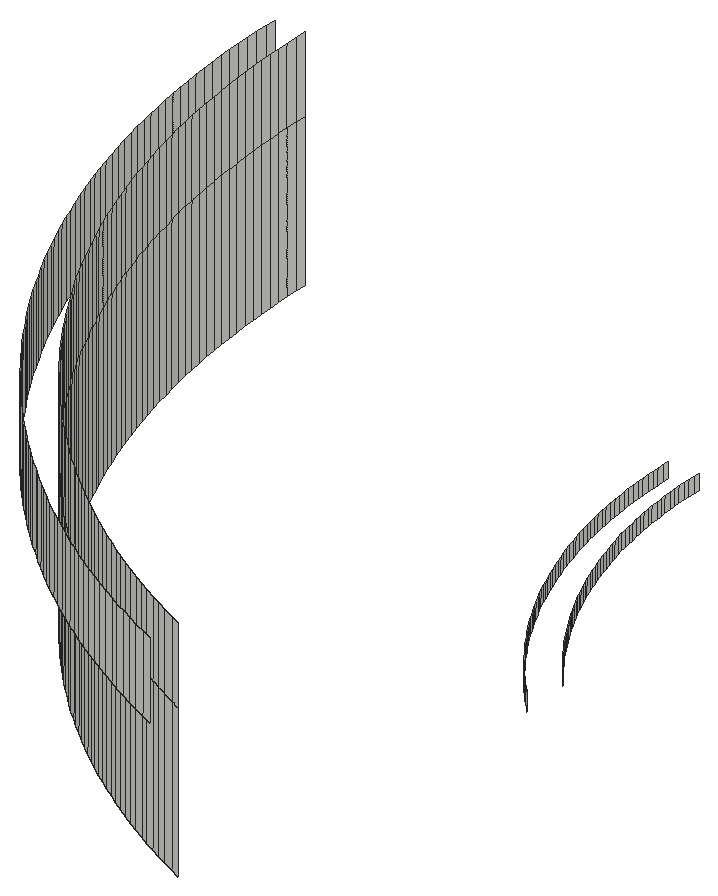
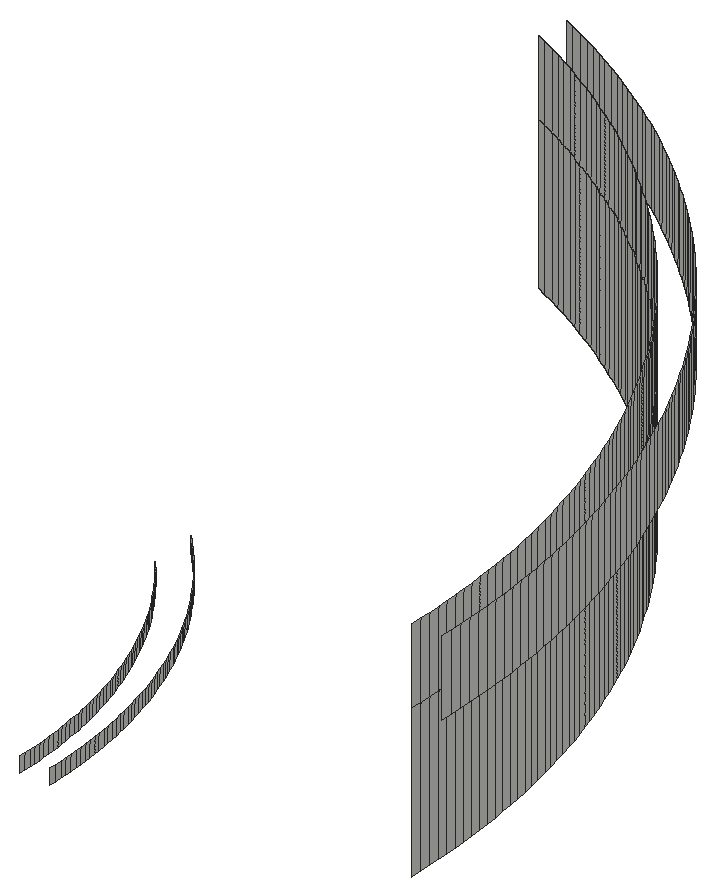
# SketchUp Ruby script. Lengths in inches.
U = 1.inch
M = Sketchup.active_model
def pt(a) = Geom::Point3d.new(a.map { |v| v * U })
def face(e, loops, mat)
  f = e.add_face(loops[0].map { |a| pt(a) })
  loops[1..].each { |l| e.add_face(l.map { |a| pt(a) }).erase! }
  f.material = f.back_material = mat if mat
  f
end
# faces: each face lists its corners as indices into pts; further lists are holes
def faces(e, pts, list, mat = nil) = list.each { |f| face(e, (f[0].is_a?(Array) ? f : [f]).map { |l| l.map { |i| pts[i] } }, mat) }
# xy, xz, yz: faces in a plane at the given z, y or x. An outline is a flat list of corners, or four numbers for a rectangle; further outlines are holes
def ring(l) = l.size == 4 ? [[l[0], l[1]], [l[2], l[1]], [l[2], l[3]], [l[0], l[3]]] : l.each_slice(2).to_a
def flat(e, list, mat, &to3) = list.each { |f| face(e, (f[0].is_a?(Array) ? f : [f]).map { |l| ring(l).map { |u, v| to3.(u, v) } }, mat) }
def xy(e, z, list, mat = nil) = flat(e, list, mat) { |x, y| [x, y, z] }
def xz(e, y, list, mat = nil) = flat(e, list, mat) { |x, z| [x, y, z] }
def yz(e, x, list, mat = nil) = flat(e, list, mat) { |y, z| [x, y, z] }
def lines(e, pts, list) = list.each { |a, b| e.add_line(pt(pts[a]), pt(pts[b])) }
# prism: a flat outline (further loops are holes) pulled along v
def prism(e, loops, v, mat = nil)
  f = face(e, loops, mat); d = Geom::Vector3d.new(v.map { |x| x * U })
  f.pushpull(f.normal.samedirection?(d) ? d.length : -d.length)
end
def box(e, o, s, mat = nil) = prism(e, [[o, [o[0] + s[0], o[1], o[2]], [o[0] + s[0], o[1] + s[1], o[2]], [o[0], o[1] + s[1], o[2]]]], [0, 0, s[2]], mat)
def at(x, y, z, deg = 0) = Geom::Transformation.translation(pt([x, y, z])) * Geom::Transformation.rotation(ORIGIN, Z_AXIS, deg.degrees)
def axes(o, x, y, z) = Geom::Transformation.new([*x, 0, *y, 0, *z, 0, *pt(o).to_a, 1])
def part(name) = M.definitions.add(name)
# library, detail: a bought-in or finely detailed component or shape, given as its bounding box
def library(name, o, s) = part(name).tap { |d| box(d.entities, o, s) }
def detail(e, o, s) = box(e.add_group.entities, o, s)
def put(e, d, t, mat = nil) = e.add_instance(d, t).tap { |i| i.material = mat if mat }
def group(e, t, mat = nil) = e.add_group.tap { |g| g.transformation = t; g.material = mat if mat }.entities
root = M.entities
yz(root,9,[[233.61,354.5,234,357]])
yz(root,10,[[233.62,349.5,234,354.5],[233.62,354.5,234,357]])
yz(root,22,[[233.78,348,234,348.5]])
yz(root,22.01,[[233.33,348,233.55,348.5]])
yz(root,23,[[233.79,348,234,348.5]])
yz(root,23.01,[[233.37,348,233.58,348.5]])
p = [[26.82,222.14,348],[26.67,222.3,348],[26.67,222.3,348.5],[26.82,222.14,348.5],[26.52,222.46,348],[26.52,222.46,348.5],
  [26.37,222.625,348],[26.37,222.625,348.5],[26.22,222.79,348],[26.22,222.79,348.5],[26.07,222.96,348],[26.07,222.96,348.5],
  [25.93,223.13,348],[25.93,223.13,348.5],[25.79,223.3,348],[25.79,223.3,348.5],[25.65,223.48,348],[25.65,223.48,348.5],
  [25.51,223.65,348],[25.51,223.65,348.5],[25.38,223.83,348],[25.38,223.83,348.5],[25.25,224.01,348],[25.25,224.01,348.5],
  [26.57,223.93,348],[26.7,223.77,348],[26.7,223.77,348.5],[26.57,223.93,348.5],[26.43,224.09,348],[26.43,224.09,348.5],
  [25.12,224.1875,348],[25.12,224.1875,348.5],[26.31,224.26,348],[26.31,224.26,348.5],[24.99,224.37,348],[24.99,224.37,348.5],
  [26.18,224.43,348],[26.18,224.43,348.5],[24.87,224.56,348],[24.87,224.56,348.5],[26.06,224.6,348],[26.06,224.6,348.5],
  [24.74,224.74,348],[24.74,224.74,348.5],[25.93,224.77,348],[25.93,224.77,348.5],[24.62,224.93,348],[24.62,224.93,348.5],
  [25.8125,224.9375,348],[25.8125,224.9375,348.5],[24.51,225.12,348],[24.51,225.12,348.5],[25.7,225.11,348],[25.7,225.11,348.5],
  [24.39,225.31,348],[24.39,225.31,348.5],[25.58,225.29,348],[25.58,225.29,348.5],[24.28,225.5,348],[24.28,225.5,348.5],
  [25.47,225.46,348],[25.47,225.46,348.5],[24.17,225.69,348],[24.17,225.69,348.5],[25.36,225.64,348],[25.36,225.64,348.5],
  [25.25,225.82,348],[25.25,225.82,348.5],[24.06,225.89,348],[24.06,225.89,348.5],[25.14,226,348],[25.14,226,348.5],
  [23.96,226.08,348],[23.96,226.08,348.5],[25.04,226.18,348],[25.04,226.18,348.5],[23.85,226.28,348],[23.85,226.28,348.5],
  [24.9375,226.37,348],[24.9375,226.37,348.5],[23.75,226.48,348],[23.75,226.48,348.5],[24.84,226.55,348],[24.84,226.55,348.5],
  [23.66,226.68,348],[23.66,226.68,348.5],[24.74,226.74,348],[24.74,226.74,348.5],[23.5625,226.88,348],[23.5625,226.88,348.5],
  [24.65,226.92,348],[24.65,226.92,348.5],[23.47,227.09,348],[23.47,227.09,348.5],[24.56,227.11,348],[24.56,227.11,348.5],
  [23.38,227.29,348],[23.38,227.29,348.5],[24.47,227.3,348],[24.47,227.3,348.5],[23.29,227.49,348],[23.29,227.49,348.5],
  [24.38,227.49,348],[24.38,227.49,348.5],[23.21,227.7,348],[23.21,227.7,348.5],[24.3,227.68,348],[24.3,227.68,348.5],
  [23.13,227.91,348],[23.13,227.91,348.5],[24.22,227.88,348],[24.22,227.88,348.5],[23.05,228.12,348],[23.05,228.12,348.5],
  [24.14,228.07,348],[24.14,228.07,348.5],[22.98,228.33,348],[22.98,228.33,348.5],[24.0625,228.27,348],[24.0625,228.27,348.5],
  [22.9,228.54,348],[22.9,228.54,348.5],[23.99,228.46,348],[23.99,228.46,348.5],[22.83,228.75,348],[22.83,228.75,348.5],
  [23.92,228.66,348],[23.92,228.66,348.5],[22.76,228.96,348],[22.76,228.96,348.5],[23.85,228.86,348],[23.85,228.86,348.5],
  [23.78,229.06,348],[23.78,229.06,348.5],[22.7,229.17,348],[22.7,229.17,348.5],[23.72,229.26,348],[23.72,229.26,348.5],
  [22.64,229.39,348],[22.64,229.39,348.5],[23.66,229.46,348],[23.66,229.46,348.5],[22.58,229.6,348],[22.58,229.6,348.5],
  [23.6,229.66,348],[23.6,229.66,348.5],[22.52,229.82,348],[22.52,229.82,348.5],[23.55,229.86,348],[23.55,229.86,348.5],
  [22.47,230.03,348],[22.47,230.03,348.5],[23.49,230.0625,348],[23.49,230.0625,348.5],[22.42,230.25,348],[22.42,230.25,348.5],
  [23.44,230.26,348],[23.44,230.26,348.5],[22.37,230.47,348],[22.37,230.47,348.5],[23.39,230.47,348],[23.39,230.47,348.5],
  [22.33,230.68,348],[22.33,230.68,348.5],[23.35,230.67,348],[23.35,230.67,348.5],[22.28,230.9,348],[22.28,230.9,348.5],
  [23.31,230.88,348],[23.31,230.88,348.5],[22.25,231.12,348],[22.25,231.12,348.5],[23.27,231.08,348],[23.27,231.08,348.5],
  [22.21,231.34,348],[22.21,231.34,348.5],[23.23,231.29,348],[23.23,231.29,348.5],[22.18,231.5625,348],[22.18,231.5625,348.5],
  [23.2,231.5,348],[23.2,231.5,348.5],[23.17,231.7,348],[23.17,231.7,348.5],[22.15,231.78,348],[22.15,231.78,348.5],
  [23.14,231.91,348],[23.14,231.91,348.5],[22.12,232,348],[22.12,232,348.5],[23.11,232.12,348],[23.11,232.12,348.5],
  [22.09,232.22,348],[22.09,232.22,348.5],[23.09,232.33,348],[23.09,232.33,348.5],[22.07,232.44,348],[22.07,232.44,348.5],
  [23.07,232.54,348],[23.07,232.54,348.5],[22.05,232.67,348],[22.05,232.67,348.5],[23.05,232.74,348],[23.05,232.74,348.5],
  [22.04,232.89,348],[22.04,232.89,348.5],[23.03,232.95,348],[23.03,232.95,348.5],[22.02,233.11,348],[22.02,233.11,348.5],
  [23.02,233.16,348],[23.02,233.16,348.5],[22.01,233.33,348],[22.01,233.33,348.5],[23.01,233.37,348],[23.01,233.37,348.5],
  [22.01,233.55,348],[22,233.78,348],[22,233.78,348.5],[22.01,233.55,348.5],[23,233.79,348],[23.01,233.58,348],
  [23.01,233.58,348.5],[23,233.79,348.5],[26.52,207.83,349.5],[26.86,207.66,349.5],[26.86,207.66,354.5],[26.52,207.83,354.5],
  [26.17,207.99,349.5],[26.17,207.99,354.5],[25.83,208.16,349.5],[25.83,208.16,354.5],[25.5,208.34,349.5],[25.5,208.34,354.5],
  [25.16,208.51,349.5],[25.16,208.51,354.5],[24.83,208.7,349.5],[24.83,208.7,354.5],[24.5,208.89,349.5],[24.5,208.89,354.5],
  [24.17,209.08,349.5],[24.17,209.08,354.5],[23.85,209.27,349.5],[23.85,209.27,354.5],[23.53,209.47,349.5],[23.53,209.47,354.5],
  [23.21,209.68,349.5],[23.21,209.68,354.5],[22.89,209.89,349.5],[22.89,209.89,354.5],[22.57,210.1,349.5],[22.57,210.1,354.5],
  [22.26,210.32,349.5],[22.26,210.32,354.5],[21.95,210.54,349.5],[21.95,210.54,354.5],[21.65,210.76,349.5],[21.65,210.76,354.5],
  [21.35,210.99,349.5],[21.35,210.99,354.5],[21.05,211.23,349.5],[21.05,211.23,354.5],[20.75,211.46,349.5],[20.75,211.46,354.5],
  [20.46,211.7,349.5],[20.46,211.7,354.5],[20.17,211.95,349.5],[20.17,211.95,354.5],[19.88,212.2,349.5],[19.88,212.2,354.5],
  [19.6,212.45,349.5],[19.6,212.45,354.5],[19.31,212.7,349.5],[19.31,212.7,354.5],[19.04,212.96,349.5],[19.04,212.96,354.5],
  [18.76,213.23,349.5],[18.76,213.23,354.5],[18.49,213.49,349.5],[18.49,213.49,354.5],[18.23,213.76,349.5],[18.23,213.76,354.5],
  [17.96,214.04,349.5],[17.96,214.04,354.5],[17.7,214.31,349.5],[17.7,214.31,354.5],[17.45,214.6,349.5],[17.45,214.6,354.5],
  [17.2,214.88,349.5],[17.2,214.88,354.5],[16.95,215.17,349.5],[16.95,215.17,354.5],[16.7,215.46,349.5],[16.7,215.46,354.5],
  [16.46,215.75,349.5],[16.46,215.75,354.5],[16.23,216.05,349.5],[16.23,216.05,354.5],[15.99,216.35,349.5],[15.99,216.35,354.5],
  [15.76,216.65,349.5],[15.76,216.65,354.5],[15.54,216.95,349.5],[15.54,216.95,354.5],[15.32,217.26,349.5],[15.32,217.26,354.5],
  [15.1,217.57,349.5],[15.1,217.57,354.5],[14.89,217.89,349.5],[14.89,217.89,354.5],[14.68,218.21,349.5],[14.68,218.21,354.5],
  [14.47,218.53,349.5],[14.47,218.53,354.5],[14.27,218.85,349.5],[14.27,218.85,354.5],[14.08,219.17,349.5],[14.08,219.17,354.5],
  [13.89,219.5,349.5],[13.89,219.5,354.5],[13.7,219.83,349.5],[13.7,219.83,354.5],[13.51,220.16,349.5],[13.51,220.16,354.5],
  [13.34,220.5,349.5],[13.34,220.5,354.5],[13.16,220.83,349.5],[13.16,220.83,354.5],[12.99,221.17,349.5],[12.99,221.17,354.5],
  [12.83,221.52,349.5],[12.83,221.52,354.5],[12.66,221.86,349.5],[12.66,221.86,354.5],[12.51,222.2,349.5],[12.51,222.2,354.5],
  [12.36,222.55,349.5],[12.36,222.55,354.5],[12.21,222.9,349.5],[12.21,222.9,354.5],[12.06,223.25,349.5],[12.06,223.25,354.5],
  [11.93,223.61,349.5],[11.93,223.61,354.5],[11.79,223.96,349.5],[11.79,223.96,354.5],[11.66,224.32,349.5],[11.66,224.32,354.5],
  [11.54,224.68,349.5],[11.54,224.68,354.5],[11.42,225.04,349.5],[11.42,225.04,354.5],[11.3,225.4,349.5],[11.3,225.4,354.5],
  [11.19,225.76,349.5],[11.19,225.76,354.5],[11.09,226.13,349.5],[11.09,226.13,354.5],[10.99,226.49,349.5],[10.99,226.49,354.5],
  [10.89,226.86,349.5],[10.89,226.86,354.5],[10.8,227.23,349.5],[10.8,227.23,354.5],[10.72,227.6,349.5],[10.72,227.6,354.5],
  [10.63,227.97,349.5],[10.63,227.97,354.5],[10.56,228.34,349.5],[10.56,228.34,354.5],[10.49,228.72,349.5],[10.49,228.72,354.5],
  [10.42,229.09,349.5],[10.42,229.09,354.5],[10.36,229.46,349.5],[10.36,229.46,354.5],[10.3,229.84,349.5],[10.3,229.84,354.5],
  [10.25,230.21,349.5],[10.25,230.21,354.5],[10.2,230.59,349.5],[10.2,230.59,354.5],[10.16,230.97,349.5],[10.16,230.97,354.5],
  [10.12,231.35,349.5],[10.12,231.35,354.5],[10.09,231.72,349.5],[10.09,231.72,354.5],[10.0625,232.1,349.5],[10.0625,232.1,354.5],
  [10.04,232.48,349.5],[10.04,232.48,354.5],[10.02,232.86,349.5],[10.02,232.86,354.5],[10.01,233.24,349.5],[10.01,233.24,354.5],
  [10,233.62,349.5],[10,233.62,354.5],[26.44,206.76,354.5],[26.8,206.59,354.5],[26.8,206.59,357],[26.44,206.76,357],
  [26.08,206.92,354.5],[26.08,206.92,357],[25.73,207.09,354.5],[25.73,207.09,357],[25.38,207.27,354.5],[25.38,207.27,357],
  [25.03,207.45,354.5],[25.03,207.45,357],[24.69,207.64,354.5],[24.69,207.64,357],[24.34,207.83,354.5],[24.34,207.83,357],
  [26.52,207.83,357],[26.86,207.66,357],[24,208.02,354.5],[24,208.02,357],[26.17,207.99,357],[23.66,208.22,354.5],
  [23.66,208.22,357],[25.83,208.16,357],[23.33,208.42,354.5],[23.33,208.42,357],[25.5,208.34,357],[25.16,208.51,357],
  [22.99,208.63,354.5],[22.99,208.63,357],[24.83,208.7,357],[22.66,208.84,354.5],[22.66,208.84,357],[24.5,208.89,357],
  [22.33,209.06,354.5],[22.33,209.06,357],[24.17,209.08,357],[22.01,209.28,354.5],[22.01,209.28,357],[23.85,209.27,357],
  [21.6875,209.5,354.5],[21.6875,209.5,357],[23.53,209.47,357],[21.37,209.73,354.5],[21.37,209.73,357],[23.21,209.68,357],
  [21.05,209.96,354.5],[21.05,209.96,357],[22.89,209.89,357],[22.57,210.1,357],[20.74,210.2,354.5],[20.74,210.2,357],
  [22.26,210.32,357],[20.43,210.44,354.5],[20.43,210.44,357],[21.95,210.54,357],[20.12,210.6875,354.5],[20.12,210.6875,357],
  [21.65,210.76,357],[19.82,210.93,354.5],[19.82,210.93,357],[21.35,210.99,357],[19.52,211.1875,354.5],[19.52,211.1875,357],
  [21.05,211.23,357],[19.22,211.44,354.5],[19.22,211.44,357],[20.75,211.46,357],[18.93,211.71,354.5],[18.93,211.71,357],
  [20.46,211.7,357],[18.64,211.97,354.5],[18.64,211.97,357],[20.17,211.95,357],[19.88,212.2,357],[18.35,212.24,354.5],
  [18.35,212.24,357],[18.07,212.51,354.5],[18.07,212.51,357],[19.6,212.45,357],[19.31,212.7,357],[17.79,212.79,354.5],
  [17.79,212.79,357],[19.04,212.96,357],[17.51,213.07,354.5],[17.51,213.07,357],[18.76,213.23,357],[17.24,213.35,354.5],
  [17.24,213.35,357],[18.49,213.49,357],[16.97,213.64,354.5],[16.97,213.64,357],[18.23,213.76,357],[16.71,213.93,354.5],
  [16.71,213.93,357],[17.96,214.04,357],[16.44,214.22,354.5],[16.44,214.22,357],[17.7,214.31,357],[16.1875,214.52,354.5],
  [16.1875,214.52,357],[17.45,214.6,357],[15.93,214.82,354.5],[15.93,214.82,357],[17.2,214.88,357],[15.6875,215.12,354.5],
  [15.6875,215.12,357],[16.95,215.17,357],[15.44,215.43,354.5],[15.44,215.43,357],[16.7,215.46,357],[15.2,215.74,354.5],
  [15.2,215.74,357],[16.46,215.75,357],[14.96,216.05,354.5],[14.96,216.05,357],[16.23,216.05,357],[15.99,216.35,357],
  [14.73,216.37,354.5],[14.73,216.37,357],[15.76,216.65,357],[14.5,216.6875,354.5],[14.5,216.6875,357],[15.54,216.95,357],
  [14.28,217.01,354.5],[14.28,217.01,357],[14.06,217.33,354.5],[14.06,217.33,357],[15.32,217.26,357],[13.84,217.66,354.5],
  [13.84,217.66,357],[15.1,217.57,357],[14.89,217.89,357],[13.63,217.99,354.5],[13.63,217.99,357],[14.68,218.21,357],
  [13.42,218.33,354.5],[13.42,218.33,357],[14.47,218.53,357],[13.22,218.66,354.5],[13.22,218.66,357],[14.27,218.85,357],
  [13.02,219,354.5],[13.02,219,357],[14.08,219.17,357],[12.83,219.34,354.5],[12.83,219.34,357],[13.89,219.5,357],
  [12.64,219.69,354.5],[12.64,219.69,357],[13.7,219.83,357],[12.45,220.03,354.5],[12.45,220.03,357],[13.51,220.16,357],
  [12.27,220.38,354.5],[12.27,220.38,357],[13.34,220.5,357],[12.09,220.73,354.5],[12.09,220.73,357],[13.16,220.83,357],
  [11.92,221.08,354.5],[11.92,221.08,357],[12.99,221.17,357],[11.76,221.44,354.5],[11.76,221.44,357],[12.83,221.52,357],
  [11.59,221.8,354.5],[11.59,221.8,357],[12.66,221.86,357],[11.4375,222.16,354.5],[11.4375,222.16,357],[12.51,222.2,357],
  [11.28,222.52,354.5],[11.28,222.52,357],[12.36,222.55,357],[11.14,222.88,354.5],[11.14,222.88,357],[12.21,222.9,357],
  [10.99,223.25,354.5],[10.99,223.25,357],[12.06,223.25,357],[10.85,223.62,354.5],[10.85,223.62,357],[11.93,223.61,357],
  [10.72,223.99,354.5],[10.72,223.99,357],[11.79,223.96,357],[10.59,224.36,354.5],[10.59,224.36,357],[11.66,224.32,357],
  [11.54,224.68,357],[10.47,224.73,354.5],[10.47,224.73,357],[10.35,225.1,354.5],[10.35,225.1,357],[11.42,225.04,357],
  [11.3,225.4,357],[10.24,225.48,354.5],[10.24,225.48,357],[11.19,225.76,357],[10.125,225.86,354.5],[10.125,225.86,357],
  [11.09,226.13,357],[10.02,226.24,354.5],[10.02,226.24,357],[10.99,226.49,357],[9.92,226.62,354.5],[9.92,226.62,357],
  [10.89,226.86,357],[9.83,227,354.5],[9.83,227,357],[10.8,227.23,357],[9.74,227.38,354.5],[9.74,227.38,357],
  [10.72,227.6,357],[9.66,227.76,354.5],[9.66,227.76,357],[10.63,227.97,357],[9.58,228.15,354.5],[9.58,228.15,357],
  [10.56,228.34,357],[9.5,228.53,354.5],[9.5,228.53,357],[10.49,228.72,357],[9.43,228.92,354.5],[9.43,228.92,357],
  [10.42,229.09,357],[9.37,229.31,354.5],[9.37,229.31,357],[10.36,229.46,357],[9.31,229.7,354.5],[9.31,229.7,357],
  [10.3,229.84,357],[9.26,230.08,354.5],[9.26,230.08,357],[10.25,230.21,357],[9.21,230.47,354.5],[9.21,230.47,357],
  [10.2,230.59,357],[9.16,230.86,354.5],[9.16,230.86,357],[10.16,230.97,357],[9.125,231.25,354.5],[9.125,231.25,357],
  [10.12,231.35,357],[9.09,231.65,354.5],[9.09,231.65,357],[10.09,231.72,357],[9.0625,232.04,354.5],[9.0625,232.04,357],
  [10.0625,232.1,357],[9.04,232.43,354.5],[9.04,232.43,357],[10.04,232.48,357],[9.02,232.82,354.5],[9.02,232.82,357],
  [10.02,232.86,357],[9.01,233.21,354.5],[9.01,233.21,357],[10.01,233.24,357],[9,233.61,354.5],[9,233.61,357],
  [10,233.62,357]]
faces(root,p,[[0,1,2,3],[1,4,5,2],[4,6,7,5],[6,8,9,7],[8,10,11,9],[10,12,13,11],[12,14,15,13],[14,16,17,15],
  [16,18,19,17],[18,20,21,19],[20,22,23,21],[24,25,26,27],[28,24,27,29],[22,30,31,23],[32,28,29,33],[30,34,35,31],
  [36,32,33,37],[34,38,39,35],[40,36,37,41],[38,42,43,39],[44,40,41,45],[42,46,47,43],[48,44,45,49],[46,50,51,47],
  [52,48,49,53],[50,54,55,51],[56,52,53,57],[54,58,59,55],[60,56,57,61],[58,62,63,59],[64,60,61,65],[66,64,65,67],
  [62,68,69,63],[70,66,67,71],[68,72,73,69],[74,70,71,75],[72,76,77,73],[78,74,75,79],[76,80,81,77],[82,78,79,83],
  [80,84,85,81],[86,82,83,87],[84,88,89,85],[90,86,87,91],[88,92,93,89],[94,90,91,95],[92,96,97,93],[98,94,95,99],
  [96,100,101,97],[102,98,99,103],[100,104,105,101],[106,102,103,107],[104,108,109,105],[110,106,107,111],[108,112,113,109],[114,110,111,115],
  [112,116,117,113],[118,114,115,119],[116,120,121,117],[122,118,119,123],[120,124,125,121],[126,122,123,127],[124,128,129,125],[130,126,127,131],
  [132,130,131,133],[128,134,135,129],[136,132,133,137],[134,138,139,135],[140,136,137,141],[138,142,143,139],[144,140,141,145],[142,146,147,143],
  [148,144,145,149],[146,150,151,147],[152,148,149,153],[150,154,155,151],[156,152,153,157],[154,158,159,155],[160,156,157,161],[158,162,163,159],
  [164,160,161,165],[162,166,167,163],[168,164,165,169],[166,170,171,167],[172,168,169,173],[170,174,175,171],[176,172,173,177],[174,178,179,175],
  [180,176,177,181],[182,180,181,183],[178,184,185,179],[186,182,183,187],[184,188,189,185],[190,186,187,191],[188,192,193,189],[194,190,191,195],
  [192,196,197,193],[198,194,195,199],[196,200,201,197],[202,198,199,203],[200,204,205,201],[206,202,203,207],[204,208,209,205],[210,206,207,211],
  [208,212,213,209],[214,210,211,215],[216,217,218,219],[220,221,222,223],[224,225,226,227],[228,224,227,229],[230,228,229,231],[232,230,231,233],
  [234,232,233,235],[236,234,235,237],[238,236,237,239],[240,238,239,241],[242,240,241,243],[244,242,243,245],[246,244,245,247],[248,246,247,249],
  [250,248,249,251],[252,250,251,253],[254,252,253,255],[256,254,255,257],[258,256,257,259],[260,258,259,261],[262,260,261,263],[264,262,263,265],
  [266,264,265,267],[268,266,267,269],[270,268,269,271],[272,270,271,273],[274,272,273,275],[276,274,275,277],[278,276,277,279],[280,278,279,281],
  [282,280,281,283],[284,282,283,285],[286,284,285,287],[288,286,287,289],[290,288,289,291],[292,290,291,293],[294,292,293,295],[296,294,295,297],
  [298,296,297,299],[300,298,299,301],[302,300,301,303],[304,302,303,305],[306,304,305,307],[308,306,307,309],[310,308,309,311],[312,310,311,313],
  [314,312,313,315],[316,314,315,317],[318,316,317,319],[320,318,319,321],[322,320,321,323],[324,322,323,325],[326,324,325,327],[328,326,327,329],
  [330,328,329,331],[332,330,331,333],[334,332,333,335],[336,334,335,337],[338,336,337,339],[340,338,339,341],[342,340,341,343],[344,342,343,345],
  [346,344,345,347],[348,346,347,349],[350,348,349,351],[352,350,351,353],[354,352,353,355],[356,354,355,357],[358,356,357,359],[360,358,359,361],
  [362,360,361,363],[364,362,363,365],[366,364,365,367],[368,366,367,369],[370,368,369,371],[372,370,371,373],[374,372,373,375],[376,374,375,377],
  [378,376,377,379],[380,378,379,381],[382,380,381,383],[384,382,383,385],[386,384,385,387],[388,386,387,389],[390,388,389,391],[392,390,391,393],
  [394,392,393,395],[396,394,395,397],[398,399,400,401],[402,398,401,403],[404,402,403,405],[406,404,405,407],[408,406,407,409],[410,408,409,411],
  [412,410,411,413],[226,227,414,415],[416,412,413,417],[227,229,418,414],[419,416,417,420],[229,231,421,418],[422,419,420,423],[231,233,424,421],
  [233,235,425,424],[426,422,423,427],[235,237,428,425],[429,426,427,430],[237,239,431,428],[432,429,430,433],[239,241,434,431],[435,432,433,436],
  [241,243,437,434],[438,435,436,439],[243,245,440,437],[441,438,439,442],[245,247,443,440],[444,441,442,445],[247,249,446,443],[249,251,447,446],
  [448,444,445,449],[251,253,450,447],[451,448,449,452],[253,255,453,450],[454,451,452,455],[255,257,456,453],[457,454,455,458],[257,259,459,456],
  [460,457,458,461],[259,261,462,459],[463,460,461,464],[261,263,465,462],[466,463,464,467],[263,265,468,465],[469,466,467,470],[265,267,471,468],
  [267,269,472,471],[473,469,470,474],[475,473,474,476],[269,271,477,472],[271,273,478,477],[479,475,476,480],[273,275,481,478],[482,479,480,483],
  [275,277,484,481],[485,482,483,486],[277,279,487,484],[488,485,486,489],[279,281,490,487],[491,488,489,492],[281,283,493,490],[494,491,492,495],
  [283,285,496,493],[497,494,495,498],[285,287,499,496],[500,497,498,501],[287,289,502,499],[503,500,501,504],[289,291,505,502],[506,503,504,507],
  [291,293,508,505],[509,506,507,510],[293,295,511,508],[512,509,510,513],[295,297,514,511],[297,299,515,514],[516,512,513,517],[299,301,518,515],
  [519,516,517,520],[301,303,521,518],[522,519,520,523],[524,522,523,525],[303,305,526,521],[527,524,525,528],[305,307,529,526],[307,309,530,529],
  [531,527,528,532],[309,311,533,530],[534,531,532,535],[311,313,536,533],[537,534,535,538],[313,315,539,536],[540,537,538,541],[315,317,542,539],
  [543,540,541,544],[317,319,545,542],[546,543,544,547],[319,321,548,545],[549,546,547,550],[321,323,551,548],[552,549,550,553],[323,325,554,551],
  [555,552,553,556],[325,327,557,554],[558,555,556,559],[327,329,560,557],[561,558,559,562],[329,331,563,560],[564,561,562,565],[331,333,566,563],
  [567,564,565,568],[333,335,569,566],[570,567,568,571],[335,337,572,569],[573,570,571,574],[337,339,575,572],[576,573,574,577],[339,341,578,575],
  [579,576,577,580],[341,343,581,578],[582,579,580,583],[343,345,584,581],[585,582,583,586],[345,347,587,584],[347,349,588,587],[589,585,586,590],
  [591,589,590,592],[349,351,593,588],[351,353,594,593],[595,591,592,596],[353,355,597,594],[598,595,596,599],[355,357,600,597],[601,598,599,602],
  [357,359,603,600],[604,601,602,605],[359,361,606,603],[607,604,605,608],[361,363,609,606],[610,607,608,611],[363,365,612,609],[613,610,611,614],
  [365,367,615,612],[616,613,614,617],[367,369,618,615],[619,616,617,620],[369,371,621,618],[622,619,620,623],[371,373,624,621],[625,622,623,626],
  [373,375,627,624],[628,625,626,629],[375,377,630,627],[631,628,629,632],[377,379,633,630],[634,631,632,635],[379,381,636,633],[637,634,635,638],
  [381,383,639,636],[640,637,638,641],[383,385,642,639],[643,640,641,644],[385,387,645,642],[646,643,644,647],[387,389,648,645],[649,646,647,650],
  [389,391,651,648],[652,649,650,653],[391,393,654,651],[655,652,653,656],[393,395,657,654],[658,655,656,659],[395,397,660,657]])
